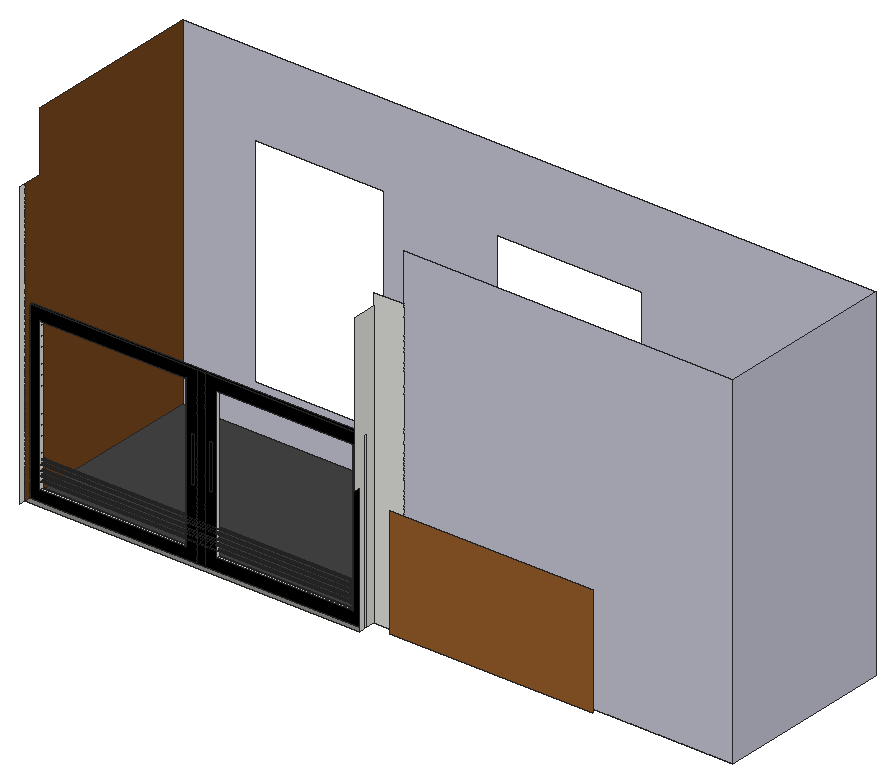
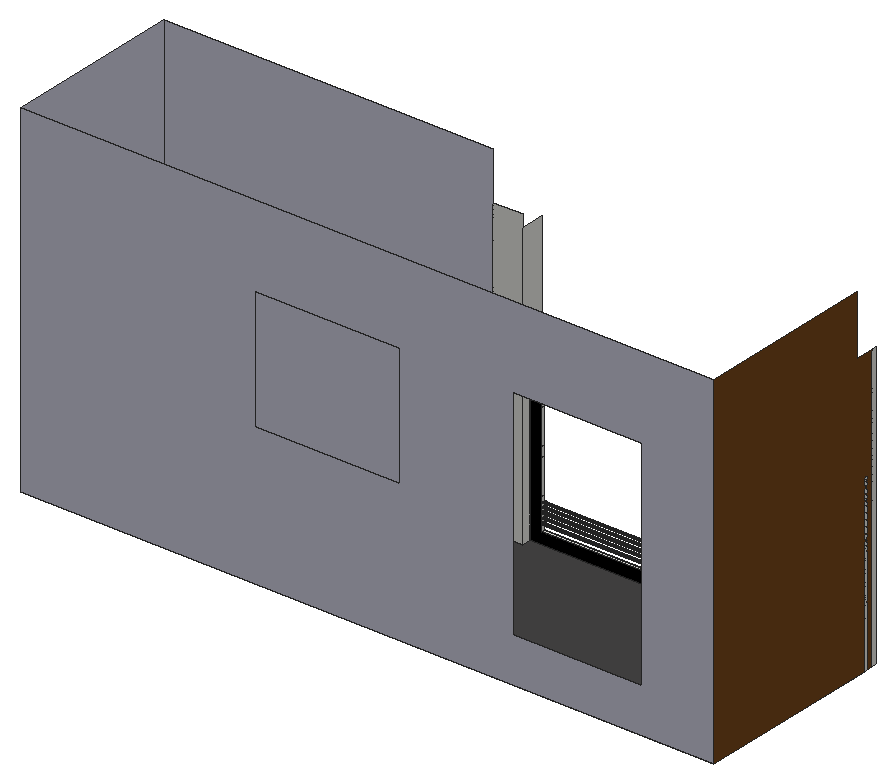
# SketchUp Ruby script. Lengths in inches.
U = 1.inch
M = Sketchup.active_model
def pt(a) = Geom::Point3d.new(a.map { |v| v * U })
def face(e, loops, mat)
  f = e.add_face(loops[0].map { |a| pt(a) })
  loops[1..].each { |l| e.add_face(l.map { |a| pt(a) }).erase! }
  f.material = f.back_material = mat if mat
  f
end
# faces: each face lists its corners as indices into pts; further lists are holes
def faces(e, pts, list, mat = nil) = list.each { |f| face(e, (f[0].is_a?(Array) ? f : [f]).map { |l| l.map { |i| pts[i] } }, mat) }
# xy, xz, yz: faces in a plane at the given z, y or x. An outline is a flat list of corners, or four numbers for a rectangle; further outlines are holes
def ring(l) = l.size == 4 ? [[l[0], l[1]], [l[2], l[1]], [l[2], l[3]], [l[0], l[3]]] : l.each_slice(2).to_a
def flat(e, list, mat, &to3) = list.each { |f| face(e, (f[0].is_a?(Array) ? f : [f]).map { |l| ring(l).map { |u, v| to3.(u, v) } }, mat) }
def xy(e, z, list, mat = nil) = flat(e, list, mat) { |x, y| [x, y, z] }
def xz(e, y, list, mat = nil) = flat(e, list, mat) { |x, z| [x, y, z] }
def yz(e, x, list, mat = nil) = flat(e, list, mat) { |y, z| [x, y, z] }
def lines(e, pts, list) = list.each { |a, b| e.add_line(pt(pts[a]), pt(pts[b])) }
# prism: a flat outline (further loops are holes) pulled along v
def prism(e, loops, v, mat = nil)
  f = face(e, loops, mat); d = Geom::Vector3d.new(v.map { |x| x * U })
  f.pushpull(f.normal.samedirection?(d) ? d.length : -d.length)
end
def box(e, o, s, mat = nil) = prism(e, [[o, [o[0] + s[0], o[1], o[2]], [o[0] + s[0], o[1] + s[1], o[2]], [o[0], o[1] + s[1], o[2]]]], [0, 0, s[2]], mat)
def at(x, y, z, deg = 0) = Geom::Transformation.translation(pt([x, y, z])) * Geom::Transformation.rotation(ORIGIN, Z_AXIS, deg.degrees)
def axes(o, x, y, z) = Geom::Transformation.new([*x, 0, *y, 0, *z, 0, *pt(o).to_a, 1])
def part(name) = M.definitions.add(name)
# library, detail: a bought-in or finely detailed component or shape, given as its bounding box
def library(name, o, s) = part(name).tap { |d| box(d.entities, o, s) }
def detail(e, o, s) = box(e.add_group.entities, o, s)
def put(e, d, t, mat = nil) = e.add_instance(d, t).tap { |i| i.material = mat if mat }
def group(e, t, mat = nil) = e.add_group.tap { |g| g.transformation = t; g.material = mat if mat }.entities
root = M.entities
M.materials.add("[0116_Lavender]").color = [199, 199, 216]
M.materials.add("[0137_Black]").color = [0, 0, 0]
M.materials.add("[Granite Dark Gray]").color = [69, 68, 68]
M.materials.add("[Granite Light Gray]").color = [132, 131, 128]
M.materials.add("[Wood Bamboo]").color = [114, 68, 27]
M.materials.add("[Wood Floor Dark]").color = [153, 94, 42]
xy(root,42,[[468,71.03,1140,78]])
xy(root,42,[[468,78,1140,78,1140,96,1860,96,1860,455.71,468,455.71]],"[Granite Dark Gray]")
xy(root,42,[[468,60,1140,71.03]],"[Granite Light Gray]")
xy(root,63.6,[[489.6,71.03,782.4,78]])
xy(root,65.95,[[843.34,71.03,1116.05,78]])
xz(root,60,[[1200,60,1608,280.8]],"[Wood Floor Dark]")
xz(root,71.03,[[[468,42,804,390],[489.6,63.6,782.4,368.4],[791.39,180.6,799.64,271.47]],[804,42,819.39,390],[[819.39,42,1140,390],[843.34,65.95,1116.05,366.05],[827.39,180.6,835.64,271.47]]],"[0137_Black]")
xz(root,78,[[[468,42,1140,390],[489.6,63.6,782.4,368.4],[843.34,65.95,1116.05,366.05]]],"[0137_Black]")
xz(root,96,[[1140,42,1200,636]])
xz(root,96,[[1200,42,1860,732]],"[0116_Lavender]")
xz(root,455.71,[[[468,42,1860,732],[611.72,132,872.28,567.56],[1098.44,324.3,1390.19,567.56]]],"[0116_Lavender]")
yz(root,468,[[48,42,60,612],[71.03,42,78,390]])
yz(root,468,[[60,42,71.03,42,71.03,390,78,390,78,42,455.71,42,455.71,732,96,732,96,612,60,612]],"[Wood Bamboo]")
yz(root,489.6,[[[71.03,63.6,78,368.4],[74.52,356.6875,74,356.75,73.52,356.95,73.1,357.27,72.78,357.6875,72.58,358.17,72.52,358.6875,72.58,359.2,72.78,359.6875,73.1,360.1,73.52,360.42,74,360.62,74.52,360.6875,75.03,360.62,75.52,360.42,75.93,360.1,76.25,359.6875,76.45,359.2,76.52,358.6875,76.45,358.17,76.25,357.6875,75.93,357.27,75.52,356.95,75.03,356.75],[74.52,346.6875,74,346.75,73.52,346.95,73.1,347.27,72.78,347.6875,72.58,348.17,72.52,348.6875,72.58,349.2,72.78,349.6875,73.1,350.1,73.52,350.42,74,350.62,74.52,350.6875,75.03,350.62,75.52,350.42,75.93,350.1,76.25,349.6875,76.45,349.2,76.52,348.6875,76.45,348.17,76.25,347.6875,75.93,347.27,75.52,346.95,75.03,346.75],[74.52,336.6875,74,336.75,73.52,336.95,73.1,337.27,72.78,337.6875,72.58,338.17,72.52,338.6875,72.58,339.2,72.78,339.6875,73.1,340.1,73.52,340.42,74,340.62,74.52,340.6875,75.03,340.62,75.52,340.42,75.93,340.1,76.25,339.6875,76.45,339.2,76.52,338.6875,76.45,338.17,76.25,337.6875,75.93,337.27,75.52,336.95,75.03,336.75],[74.52,326.6875,74,326.75,73.52,326.95,73.1,327.27,72.78,327.6875,72.58,328.17,72.52,328.6875,72.58,329.2,72.78,329.6875,73.1,330.1,73.52,330.42,74,330.62,74.52,330.6875,75.03,330.62,75.52,330.42,75.93,330.1,76.25,329.6875,76.45,329.2,76.52,328.6875,76.45,328.17,76.25,327.6875,75.93,327.27,75.52,326.95,75.03,326.75],[74.52,316.6875,74,316.75,73.52,316.95,73.1,317.27,72.78,317.6875,72.58,318.17,72.52,318.6875,72.58,319.2,72.78,319.6875,73.1,320.1,73.52,320.42,74,320.62,74.52,320.6875,75.03,320.62,75.52,320.42,75.93,320.1,76.25,319.6875,76.45,319.2,76.52,318.6875,76.45,318.17,76.25,317.6875,75.93,317.27,75.52,316.95,75.03,316.75],[74.52,306.6875,74,306.75,73.52,306.95,73.1,307.27,72.78,307.6875,72.58,308.17,72.52,308.6875,72.58,309.2,72.78,309.6875,73.1,310.1,73.52,310.42,74,310.62,74.52,310.6875,75.03,310.62,75.52,310.42,75.93,310.1,76.25,309.6875,76.45,309.2,76.52,308.6875,76.45,308.17,76.25,307.6875,75.93,307.27,75.52,306.95,75.03,306.75],[74.52,296.6875,74,296.75,73.52,296.95,73.1,297.27,72.78,297.6875,72.58,298.17,72.52,298.6875,72.58,299.2,72.78,299.6875,73.1,300.1,73.52,300.42,74,300.62,74.52,300.6875,75.03,300.62,75.52,300.42,75.93,300.1,76.25,299.6875,76.45,299.2,76.52,298.6875,76.45,298.17,76.25,297.6875,75.93,297.27,75.52,296.95,75.03,296.75],[74.52,286.6875,74,286.75,73.52,286.95,73.1,287.27,72.78,287.6875,72.58,288.17,72.52,288.6875,72.58,289.2,72.78,289.6875,73.1,290.1,73.52,290.42,74,290.62,74.52,290.6875,75.03,290.62,75.52,290.42,75.93,290.1,76.25,289.6875,76.45,289.2,76.52,288.6875,76.45,288.17,76.25,287.6875,75.93,287.27,75.52,286.95,75.03,286.75],[74.52,276.6875,74,276.75,73.52,276.95,73.1,277.27,72.78,277.6875,72.58,278.17,72.52,278.6875,72.58,279.2,72.78,279.6875,73.1,280.1,73.52,280.42,74,280.62,74.52,280.6875,75.03,280.62,75.52,280.42,75.93,280.1,76.25,279.6875,76.45,279.2,76.52,278.6875,76.45,278.17,76.25,277.6875,75.93,277.27,75.52,276.95,75.03,276.75],[74.52,266.6875,74,266.75,73.52,266.95,73.1,267.27,72.78,267.6875,72.58,268.17,72.52,268.6875,72.58,269.2,72.78,269.6875,73.1,270.1,73.52,270.42,74,270.62,74.52,270.6875,75.03,270.62,75.52,270.42,75.93,270.1,76.25,269.6875,76.45,269.2,76.52,268.6875,76.45,268.17,76.25,267.6875,75.93,267.27,75.52,266.95,75.03,266.75],[74.52,256.6875,74,256.75,73.52,256.95,73.1,257.27,72.78,257.6875,72.58,258.17,72.52,258.6875,72.58,259.2,72.78,259.6875,73.1,260.1,73.52,260.42,74,260.62,74.52,260.6875,75.03,260.62,75.52,260.42,75.93,260.1,76.25,259.6875,76.45,259.2,76.52,258.6875,76.45,258.17,76.25,257.6875,75.93,257.27,75.52,256.95,75.03,256.75],[74.52,246.6875,74,246.75,73.52,246.95,73.1,247.27,72.78,247.6875,72.58,248.17,72.52,248.6875,72.58,249.2,72.78,249.6875,73.1,250.1,73.52,250.42,74,250.62,74.52,250.6875,75.03,250.62,75.52,250.42,75.93,250.1,76.25,249.6875,76.45,249.2,76.52,248.6875,76.45,248.17,76.25,247.6875,75.93,247.27,75.52,246.95,75.03,246.75],[74.52,236.6875,74,236.75,73.52,236.95,73.1,237.27,72.78,237.6875,72.58,238.17,72.52,238.6875,72.58,239.2,72.78,239.6875,73.1,240.1,73.52,240.42,74,240.62,74.52,240.6875,75.03,240.62,75.52,240.42,75.93,240.1,76.25,239.6875,76.45,239.2,76.52,238.6875,76.45,238.17,76.25,237.6875,75.93,237.27,75.52,236.95,75.03,236.75],[74.52,226.6875,74,226.75,73.52,226.95,73.1,227.27,72.78,227.6875,72.58,228.17,72.52,228.6875,72.58,229.2,72.78,229.6875,73.1,230.1,73.52,230.42,74,230.62,74.52,230.6875,75.03,230.62,75.52,230.42,75.93,230.1,76.25,229.6875,76.45,229.2,76.52,228.6875,76.45,228.17,76.25,227.6875,75.93,227.27,75.52,226.95,75.03,226.75],[74.52,216.6875,74,216.75,73.52,216.95,73.1,217.27,72.78,217.6875,72.58,218.17,72.52,218.6875,72.58,219.2,72.78,219.6875,73.1,220.1,73.52,220.42,74,220.62,74.52,220.6875,75.03,220.62,75.52,220.42,75.93,220.1,76.25,219.6875,76.45,219.2,76.52,218.6875,76.45,218.17,76.25,217.6875,75.93,217.27,75.52,216.95,75.03,216.75],[74.52,206.6875,74,206.75,73.52,206.95,73.1,207.27,72.78,207.6875,72.58,208.17,72.52,208.6875,72.58,209.2,72.78,209.6875,73.1,210.1,73.52,210.42,74,210.62,74.52,210.6875,75.03,210.62,75.52,210.42,75.93,210.1,76.25,209.6875,76.45,209.2,76.52,208.6875,76.45,208.17,76.25,207.6875,75.93,207.27,75.52,206.95,75.03,206.75],[74.52,196.6875,74,196.75,73.52,196.95,73.1,197.27,72.78,197.6875,72.58,198.17,72.52,198.6875,72.58,199.2,72.78,199.6875,73.1,200.1,73.52,200.42,74,200.62,74.52,200.6875,75.03,200.62,75.52,200.42,75.93,200.1,76.25,199.6875,76.45,199.2,76.52,198.6875,76.45,198.17,76.25,197.6875,75.93,197.27,75.52,196.95,75.03,196.75],[74.52,186.6875,74,186.75,73.52,186.95,73.1,187.27,72.78,187.6875,72.58,188.17,72.52,188.6875,72.58,189.2,72.78,189.6875,73.1,190.1,73.52,190.42,74,190.62,74.52,190.6875,75.03,190.62,75.52,190.42,75.93,190.1,76.25,189.6875,76.45,189.2,76.52,188.6875,76.45,188.17,76.25,187.6875,75.93,187.27,75.52,186.95,75.03,186.75],[74.52,176.6875,74,176.75,73.52,176.95,73.1,177.27,72.78,177.6875,72.58,178.17,72.52,178.6875,72.58,179.2,72.78,179.6875,73.1,180.1,73.52,180.42,74,180.62,74.52,180.6875,75.03,180.62,75.52,180.42,75.93,180.1,76.25,179.6875,76.45,179.2,76.52,178.6875,76.45,178.17,76.25,177.6875,75.93,177.27,75.52,176.95,75.03,176.75],[74.52,166.6875,74,166.75,73.52,166.95,73.1,167.27,72.78,167.6875,72.58,168.17,72.52,168.6875,72.58,169.2,72.78,169.6875,73.1,170.1,73.52,170.42,74,170.62,74.52,170.6875,75.03,170.62,75.52,170.42,75.93,170.1,76.25,169.6875,76.45,169.2,76.52,168.6875,76.45,168.17,76.25,167.6875,75.93,167.27,75.52,166.95,75.03,166.75],[74.52,156.6875,74,156.75,73.52,156.95,73.1,157.27,72.78,157.6875,72.58,158.17,72.52,158.6875,72.58,159.2,72.78,159.6875,73.1,160.1,73.52,160.42,74,160.62,74.52,160.6875,75.03,160.62,75.52,160.42,75.93,160.1,76.25,159.6875,76.45,159.2,76.52,158.6875,76.45,158.17,76.25,157.6875,75.93,157.27,75.52,156.95,75.03,156.75],[74.52,146.6875,74,146.75,73.52,146.95,73.1,147.27,72.78,147.6875,72.58,148.17,72.52,148.6875,72.58,149.2,72.78,149.6875,73.1,150.1,73.52,150.42,74,150.62,74.52,150.6875,75.03,150.62,75.52,150.42,75.93,150.1,76.25,149.6875,76.45,149.2,76.52,148.6875,76.45,148.17,76.25,147.6875,75.93,147.27,75.52,146.95,75.03,146.75],[74.52,136.6875,74,136.75,73.52,136.95,73.1,137.27,72.78,137.6875,72.58,138.17,72.52,138.6875,72.58,139.2,72.78,139.6875,73.1,140.1,73.52,140.42,74,140.62,74.52,140.6875,75.03,140.62,75.52,140.42,75.93,140.1,76.25,139.6875,76.45,139.2,76.52,138.6875,76.45,138.17,76.25,137.6875,75.93,137.27,75.52,136.95,75.03,136.75],[74.52,126.6875,74,126.75,73.52,126.95,73.1,127.27,72.78,127.6875,72.58,128.17,72.52,128.6875,72.58,129.2,72.78,129.6875,73.1,130.1,73.52,130.42,74,130.62,74.52,130.6875,75.03,130.62,75.52,130.42,75.93,130.1,76.25,129.6875,76.45,129.2,76.52,128.6875,76.45,128.17,76.25,127.6875,75.93,127.27,75.52,126.95,75.03,126.75],[74.52,116.6875,74,116.75,73.52,116.95,73.1,117.27,72.78,117.6875,72.58,118.17,72.52,118.6875,72.58,119.2,72.78,119.6875,73.1,120.1,73.52,120.42,74,120.62,74.52,120.6875,75.03,120.62,75.52,120.42,75.93,120.1,76.25,119.6875,76.45,119.2,76.52,118.6875,76.45,118.17,76.25,117.6875,75.93,117.27,75.52,116.95,75.03,116.75],[74.52,106.6875,74,106.75,73.52,106.95,73.1,107.27,72.78,107.6875,72.58,108.17,72.52,108.6875,72.58,109.2,72.78,109.6875,73.1,110.1,73.52,110.42,74,110.62,74.52,110.6875,75.03,110.62,75.52,110.42,75.93,110.1,76.25,109.6875,76.45,109.2,76.52,108.6875,76.45,108.17,76.25,107.6875,75.93,107.27,75.52,106.95,75.03,106.75],[74.52,96.6875,74,96.75,73.52,96.95,73.1,97.27,72.78,97.6875,72.58,98.17,72.52,98.6875,72.58,99.2,72.78,99.6875,73.1,100.1,73.52,100.42,74,100.62,74.52,100.6875,75.03,100.62,75.52,100.42,75.93,100.1,76.25,99.6875,76.45,99.2,76.52,98.6875,76.45,98.17,76.25,97.6875,75.93,97.27,75.52,96.95,75.03,96.75],[74.52,86.6875,74,86.75,73.52,86.95,73.1,87.27,72.78,87.6875,72.58,88.17,72.52,88.6875,72.58,89.2,72.78,89.6875,73.1,90.1,73.52,90.42,74,90.62,74.52,90.6875,75.03,90.62,75.52,90.42,75.93,90.1,76.25,89.6875,76.45,89.2,76.52,88.6875,76.45,88.17,76.25,87.6875,75.93,87.27,75.52,86.95,75.03,86.75],[74.52,76.6875,74,76.75,73.52,76.95,73.1,77.27,72.78,77.6875,72.58,78.17,72.52,78.6875,72.58,79.2,72.78,79.6875,73.1,80.1,73.52,80.42,74,80.62,74.52,80.6875,75.03,80.62,75.52,80.42,75.93,80.1,76.25,79.6875,76.45,79.2,76.52,78.6875,76.45,78.17,76.25,77.6875,75.93,77.27,75.52,76.95,75.03,76.75]]])
yz(root,782.4,[[71.03,63.6,78,368.4]])
yz(root,843.34,[[71.03,65.95,78,366.05]])
yz(root,1116.05,[[[71.03,65.95,78,366.05],[74.52,316.6875,75.03,316.75,75.52,316.95,75.93,317.27,76.25,317.6875,76.45,318.17,76.52,318.6875,76.45,319.2,76.25,319.6875,75.93,320.1,75.52,320.42,75.03,320.62,74.52,320.6875,74,320.62,73.52,320.42,73.1,320.1,72.78,319.6875,72.58,319.2,72.52,318.6875,72.58,318.17,72.78,317.6875,73.1,317.27,73.52,316.95,74,316.75],[74.52,326.6875,75.03,326.75,75.52,326.95,75.93,327.27,76.25,327.6875,76.45,328.17,76.52,328.6875,76.45,329.2,76.25,329.6875,75.93,330.1,75.52,330.42,75.03,330.62,74.52,330.6875,74,330.62,73.52,330.42,73.1,330.1,72.78,329.6875,72.58,329.2,72.52,328.6875,72.58,328.17,72.78,327.6875,73.1,327.27,73.52,326.95,74,326.75],[74.52,346.6875,75.03,346.75,75.52,346.95,75.93,347.27,76.25,347.6875,76.45,348.17,76.52,348.6875,76.45,349.2,76.25,349.6875,75.93,350.1,75.52,350.42,75.03,350.62,74.52,350.6875,74,350.62,73.52,350.42,73.1,350.1,72.78,349.6875,72.58,349.2,72.52,348.6875,72.58,348.17,72.78,347.6875,73.1,347.27,73.52,346.95,74,346.75],[74.52,356.6875,75.03,356.75,75.52,356.95,75.93,357.27,76.25,357.6875,76.45,358.17,76.52,358.6875,76.45,359.2,76.25,359.6875,75.93,360.1,75.52,360.42,75.03,360.62,74.52,360.6875,74,360.62,73.52,360.42,73.1,360.1,72.78,359.6875,72.58,359.2,72.52,358.6875,72.58,358.17,72.78,357.6875,73.1,357.27,73.52,356.95,74,356.75],[74.52,136.6875,75.03,136.75,75.52,136.95,75.93,137.27,76.25,137.6875,76.45,138.17,76.52,138.6875,76.45,139.2,76.25,139.6875,75.93,140.1,75.52,140.42,75.03,140.62,74.52,140.6875,74,140.62,73.52,140.42,73.1,140.1,72.78,139.6875,72.58,139.2,72.52,138.6875,72.58,138.17,72.78,137.6875,73.1,137.27,73.52,136.95,74,136.75],[74.52,146.6875,75.03,146.75,75.52,146.95,75.93,147.27,76.25,147.6875,76.45,148.17,76.52,148.6875,76.45,149.2,76.25,149.6875,75.93,150.1,75.52,150.42,75.03,150.62,74.52,150.6875,74,150.62,73.52,150.42,73.1,150.1,72.78,149.6875,72.58,149.2,72.52,148.6875,72.58,148.17,72.78,147.6875,73.1,147.27,73.52,146.95,74,146.75],[74.52,156.6875,75.03,156.75,75.52,156.95,75.93,157.27,76.25,157.6875,76.45,158.17,76.52,158.6875,76.45,159.2,76.25,159.6875,75.93,160.1,75.52,160.42,75.03,160.62,74.52,160.6875,74,160.62,73.52,160.42,73.1,160.1,72.78,159.6875,72.58,159.2,72.52,158.6875,72.58,158.17,72.78,157.6875,73.1,157.27,73.52,156.95,74,156.75],[74.52,166.6875,75.03,166.75,75.52,166.95,75.93,167.27,76.25,167.6875,76.45,168.17,76.52,168.6875,76.45,169.2,76.25,169.6875,75.93,170.1,75.52,170.42,75.03,170.62,74.52,170.6875,74,170.62,73.52,170.42,73.1,170.1,72.78,169.6875,72.58,169.2,72.52,168.6875,72.58,168.17,72.78,167.6875,73.1,167.27,73.52,166.95,74,166.75],[74.52,176.6875,75.03,176.75,75.52,176.95,75.93,177.27,76.25,177.6875,76.45,178.17,76.52,178.6875,76.45,179.2,76.25,179.6875,75.93,180.1,75.52,180.42,75.03,180.62,74.52,180.6875,74,180.62,73.52,180.42,73.1,180.1,72.78,179.6875,72.58,179.2,72.52,178.6875,72.58,178.17,72.78,177.6875,73.1,177.27,73.52,176.95,74,176.75],[74.52,186.6875,75.03,186.75,75.52,186.95,75.93,187.27,76.25,187.6875,76.45,188.17,76.52,188.6875,76.45,189.2,76.25,189.6875,75.93,190.1,75.52,190.42,75.03,190.62,74.52,190.6875,74,190.62,73.52,190.42,73.1,190.1,72.78,189.6875,72.58,189.2,72.52,188.6875,72.58,188.17,72.78,187.6875,73.1,187.27,73.52,186.95,74,186.75],[74.52,196.6875,75.03,196.75,75.52,196.95,75.93,197.27,76.25,197.6875,76.45,198.17,76.52,198.6875,76.45,199.2,76.25,199.6875,75.93,200.1,75.52,200.42,75.03,200.62,74.52,200.6875,74,200.62,73.52,200.42,73.1,200.1,72.78,199.6875,72.58,199.2,72.52,198.6875,72.58,198.17,72.78,197.6875,73.1,197.27,73.52,196.95,74,196.75],[74.52,206.6875,75.03,206.75,75.52,206.95,75.93,207.27,76.25,207.6875,76.45,208.17,76.52,208.6875,76.45,209.2,76.25,209.6875,75.93,210.1,75.52,210.42,75.03,210.62,74.52,210.6875,74,210.62,73.52,210.42,73.1,210.1,72.78,209.6875,72.58,209.2,72.52,208.6875,72.58,208.17,72.78,207.6875,73.1,207.27,73.52,206.95,74,206.75],[74.52,216.6875,75.03,216.75,75.52,216.95,75.93,217.27,76.25,217.6875,76.45,218.17,76.52,218.6875,76.45,219.2,76.25,219.6875,75.93,220.1,75.52,220.42,75.03,220.62,74.52,220.6875,74,220.62,73.52,220.42,73.1,220.1,72.78,219.6875,72.58,219.2,72.52,218.6875,72.58,218.17,72.78,217.6875,73.1,217.27,73.52,216.95,74,216.75],[74.52,226.6875,75.03,226.75,75.52,226.95,75.93,227.27,76.25,227.6875,76.45,228.17,76.52,228.6875,76.45,229.2,76.25,229.6875,75.93,230.1,75.52,230.42,75.03,230.62,74.52,230.6875,74,230.62,73.52,230.42,73.1,230.1,72.78,229.6875,72.58,229.2,72.52,228.6875,72.58,228.17,72.78,227.6875,73.1,227.27,73.52,226.95,74,226.75],[74.52,236.6875,75.03,236.75,75.52,236.95,75.93,237.27,76.25,237.6875,76.45,238.17,76.52,238.6875,76.45,239.2,76.25,239.6875,75.93,240.1,75.52,240.42,75.03,240.62,74.52,240.6875,74,240.62,73.52,240.42,73.1,240.1,72.78,239.6875,72.58,239.2,72.52,238.6875,72.58,238.17,72.78,237.6875,73.1,237.27,73.52,236.95,74,236.75],[74.52,246.6875,75.03,246.75,75.52,246.95,75.93,247.27,76.25,247.6875,76.45,248.17,76.52,248.6875,76.45,249.2,76.25,249.6875,75.93,250.1,75.52,250.42,75.03,250.62,74.52,250.6875,74,250.62,73.52,250.42,73.1,250.1,72.78,249.6875,72.58,249.2,72.52,248.6875,72.58,248.17,72.78,247.6875,73.1,247.27,73.52,246.95,74,246.75],[74.52,256.6875,75.03,256.75,75.52,256.95,75.93,257.27,76.25,257.6875,76.45,258.17,76.52,258.6875,76.45,259.2,76.25,259.6875,75.93,260.1,75.52,260.42,75.03,260.62,74.52,260.6875,74,260.62,73.52,260.42,73.1,260.1,72.78,259.6875,72.58,259.2,72.52,258.6875,72.58,258.17,72.78,257.6875,73.1,257.27,73.52,256.95,74,256.75],[74.52,266.6875,75.03,266.75,75.52,266.95,75.93,267.27,76.25,267.6875,76.45,268.17,76.52,268.6875,76.45,269.2,76.25,269.6875,75.93,270.1,75.52,270.42,75.03,270.62,74.52,270.6875,74,270.62,73.52,270.42,73.1,270.1,72.78,269.6875,72.58,269.2,72.52,268.6875,72.58,268.17,72.78,267.6875,73.1,267.27,73.52,266.95,74,266.75],[74.52,276.6875,75.03,276.75,75.52,276.95,75.93,277.27,76.25,277.6875,76.45,278.17,76.52,278.6875,76.45,279.2,76.25,279.6875,75.93,280.1,75.52,280.42,75.03,280.62,74.52,280.6875,74,280.62,73.52,280.42,73.1,280.1,72.78,279.6875,72.58,279.2,72.52,278.6875,72.58,278.17,72.78,277.6875,73.1,277.27,73.52,276.95,74,276.75],[74.52,286.6875,75.03,286.75,75.52,286.95,75.93,287.27,76.25,287.6875,76.45,288.17,76.52,288.6875,76.45,289.2,76.25,289.6875,75.93,290.1,75.52,290.42,75.03,290.62,74.52,290.6875,74,290.62,73.52,290.42,73.1,290.1,72.78,289.6875,72.58,289.2,72.52,288.6875,72.58,288.17,72.78,287.6875,73.1,287.27,73.52,286.95,74,286.75],[74.52,296.6875,75.03,296.75,75.52,296.95,75.93,297.27,76.25,297.6875,76.45,298.17,76.52,298.6875,76.45,299.2,76.25,299.6875,75.93,300.1,75.52,300.42,75.03,300.62,74.52,300.6875,74,300.62,73.52,300.42,73.1,300.1,72.78,299.6875,72.58,299.2,72.52,298.6875,72.58,298.17,72.78,297.6875,73.1,297.27,73.52,296.95,74,296.75],[74.52,306.6875,75.03,306.75,75.52,306.95,75.93,307.27,76.25,307.6875,76.45,308.17,76.52,308.6875,76.45,309.2,76.25,309.6875,75.93,310.1,75.52,310.42,75.03,310.62,74.52,310.6875,74,310.62,73.52,310.42,73.1,310.1,72.78,309.6875,72.58,309.2,72.52,308.6875,72.58,308.17,72.78,307.6875,73.1,307.27,73.52,306.95,74,306.75],[74.52,126.6875,75.03,126.75,75.52,126.95,75.93,127.27,76.25,127.6875,76.45,128.17,76.52,128.6875,76.45,129.2,76.25,129.6875,75.93,130.1,75.52,130.42,75.03,130.62,74.52,130.6875,74,130.62,73.52,130.42,73.1,130.1,72.78,129.6875,72.58,129.2,72.52,128.6875,72.58,128.17,72.78,127.6875,73.1,127.27,73.52,126.95,74,126.75],[74.52,76.6875,75.03,76.75,75.52,76.95,75.93,77.27,76.25,77.6875,76.45,78.17,76.52,78.6875,76.45,79.2,76.25,79.6875,75.93,80.1,75.52,80.42,75.03,80.62,74.52,80.6875,74,80.62,73.52,80.42,73.1,80.1,72.78,79.6875,72.58,79.2,72.52,78.6875,72.58,78.17,72.78,77.6875,73.1,77.27,73.52,76.95,74,76.75],[74.52,86.6875,75.03,86.75,75.52,86.95,75.93,87.27,76.25,87.6875,76.45,88.17,76.52,88.6875,76.45,89.2,76.25,89.6875,75.93,90.1,75.52,90.42,75.03,90.62,74.52,90.6875,74,90.62,73.52,90.42,73.1,90.1,72.78,89.6875,72.58,89.2,72.52,88.6875,72.58,88.17,72.78,87.6875,73.1,87.27,73.52,86.95,74,86.75],[74.52,96.6875,75.03,96.75,75.52,96.95,75.93,97.27,76.25,97.6875,76.45,98.17,76.52,98.6875,76.45,99.2,76.25,99.6875,75.93,100.1,75.52,100.42,75.03,100.62,74.52,100.6875,74,100.62,73.52,100.42,73.1,100.1,72.78,99.6875,72.58,99.2,72.52,98.6875,72.58,98.17,72.78,97.6875,73.1,97.27,73.52,96.95,74,96.75],[74.52,106.6875,75.03,106.75,75.52,106.95,75.93,107.27,76.25,107.6875,76.45,108.17,76.52,108.6875,76.45,109.2,76.25,109.6875,75.93,110.1,75.52,110.42,75.03,110.62,74.52,110.6875,74,110.62,73.52,110.42,73.1,110.1,72.78,109.6875,72.58,109.2,72.52,108.6875,72.58,108.17,72.78,107.6875,73.1,107.27,73.52,106.95,74,106.75]]])
yz(root,1116.35,[[74.52,116.6875,75.03,116.75,75.52,116.95,75.93,117.27,76.25,117.6875,76.45,118.17,76.52,118.6875,76.45,119.2,76.25,119.6875,75.93,120.1,75.52,120.42,75.03,120.62,74.52,120.6875,74,120.62,73.52,120.42,73.1,120.1,72.78,119.6875,72.58,119.2,72.52,118.6875,72.58,118.17,72.78,117.6875,73.1,117.27,73.52,116.95,74,116.75]])
yz(root,1140,[[60,42,60,300,48,300,48,612,96,612,96,42,78,42,78,390,71.03,390,71.03,42],[71.03,42,78,390]])
yz(root,1860,[[96,42,455.71,732]],"[0116_Lavender]")
p = [[489.6,74,76.75],[489.6,74.52,76.6875],[1116.05,74.52,76.6875],[1116.05,74,76.75],[489.6,75.03,76.75],[1116.05,75.03,76.75],
  [489.6,73.52,76.95],[1116.05,73.52,76.95],[489.6,75.52,76.95],[1116.05,75.52,76.95],[489.6,73.1,77.27],[1116.05,73.1,77.27],
  [489.6,75.93,77.27],[1116.05,75.93,77.27],[489.6,72.78,77.6875],[1116.05,72.78,77.6875],[489.6,76.25,77.6875],[1116.05,76.25,77.6875],
  [489.6,72.58,78.17],[1116.05,72.58,78.17],[489.6,76.45,78.17],[1116.05,76.45,78.17],[489.6,72.52,78.6875],[1116.05,72.52,78.6875],
  [489.6,76.52,78.6875],[1116.05,76.52,78.6875],[489.6,72.58,79.2],[1116.05,72.58,79.2],[489.6,76.45,79.2],[1116.05,76.45,79.2],
  [489.6,72.78,79.6875],[1116.05,72.78,79.6875],[489.6,76.25,79.6875],[1116.05,76.25,79.6875],[489.6,73.1,80.1],[1116.05,73.1,80.1],
  [489.6,75.93,80.1],[1116.05,75.93,80.1],[489.6,73.52,80.42],[1116.05,73.52,80.42],[489.6,75.52,80.42],[1116.05,75.52,80.42],
  [489.6,74,80.62],[1116.05,74,80.62],[489.6,75.03,80.62],[1116.05,75.03,80.62],[489.6,74.52,80.6875],[1116.05,74.52,80.6875],
  [489.6,74,86.75],[489.6,74.52,86.6875],[1116.05,74.52,86.6875],[1116.05,74,86.75],[489.6,75.03,86.75],[1116.05,75.03,86.75],
  [489.6,73.52,86.95],[1116.05,73.52,86.95],[489.6,75.52,86.95],[1116.05,75.52,86.95],[489.6,73.1,87.27],[1116.05,73.1,87.27],
  [489.6,75.93,87.27],[1116.05,75.93,87.27],[489.6,72.78,87.6875],[1116.05,72.78,87.6875],[489.6,76.25,87.6875],[1116.05,76.25,87.6875],
  [489.6,72.58,88.17],[1116.05,72.58,88.17],[489.6,76.45,88.17],[1116.05,76.45,88.17],[489.6,72.52,88.6875],[1116.05,72.52,88.6875],
  [489.6,76.52,88.6875],[1116.05,76.52,88.6875],[489.6,72.58,89.2],[1116.05,72.58,89.2],[489.6,76.45,89.2],[1116.05,76.45,89.2],
  [489.6,72.78,89.6875],[1116.05,72.78,89.6875],[489.6,76.25,89.6875],[1116.05,76.25,89.6875],[489.6,73.1,90.1],[1116.05,73.1,90.1],
  [489.6,75.93,90.1],[1116.05,75.93,90.1],[489.6,73.52,90.42],[1116.05,73.52,90.42],[489.6,75.52,90.42],[1116.05,75.52,90.42],
  [489.6,74,90.62],[1116.05,74,90.62],[489.6,75.03,90.62],[1116.05,75.03,90.62],[489.6,74.52,90.6875],[1116.05,74.52,90.6875],
  [489.6,74,96.75],[489.6,74.52,96.6875],[1116.05,74.52,96.6875],[1116.05,74,96.75],[489.6,75.03,96.75],[1116.05,75.03,96.75],
  [489.6,73.52,96.95],[1116.05,73.52,96.95],[489.6,75.52,96.95],[1116.05,75.52,96.95],[489.6,73.1,97.27],[1116.05,73.1,97.27],
  [489.6,75.93,97.27],[1116.05,75.93,97.27],[489.6,72.78,97.6875],[1116.05,72.78,97.6875],[489.6,76.25,97.6875],[1116.05,76.25,97.6875],
  [489.6,72.58,98.17],[1116.05,72.58,98.17],[489.6,76.45,98.17],[1116.05,76.45,98.17],[489.6,72.52,98.6875],[1116.05,72.52,98.6875],
  [489.6,76.52,98.6875],[1116.05,76.52,98.6875],[489.6,72.58,99.2],[1116.05,72.58,99.2],[489.6,76.45,99.2],[1116.05,76.45,99.2],
  [489.6,72.78,99.6875],[1116.05,72.78,99.6875],[489.6,76.25,99.6875],[1116.05,76.25,99.6875],[489.6,73.1,100.1],[1116.05,73.1,100.1],
  [489.6,75.93,100.1],[1116.05,75.93,100.1],[489.6,73.52,100.42],[1116.05,73.52,100.42],[489.6,75.52,100.42],[1116.05,75.52,100.42],
  [489.6,74,100.62],[1116.05,74,100.62],[489.6,75.03,100.62],[1116.05,75.03,100.62],[489.6,74.52,100.6875],[1116.05,74.52,100.6875],
  [489.6,74,106.75],[489.6,74.52,106.6875],[1116.05,74.52,106.6875],[1116.05,74,106.75],[489.6,75.03,106.75],[1116.05,75.03,106.75],
  [489.6,73.52,106.95],[1116.05,73.52,106.95],[489.6,75.52,106.95],[1116.05,75.52,106.95],[489.6,73.1,107.27],[1116.05,73.1,107.27],
  [489.6,75.93,107.27],[1116.05,75.93,107.27],[489.6,72.78,107.6875],[1116.05,72.78,107.6875],[489.6,76.25,107.6875],[1116.05,76.25,107.6875],
  [489.6,72.58,108.17],[1116.05,72.58,108.17],[489.6,76.45,108.17],[1116.05,76.45,108.17],[489.6,72.52,108.6875],[1116.05,72.52,108.6875],
  [489.6,76.52,108.6875],[1116.05,76.52,108.6875],[489.6,72.58,109.2],[1116.05,72.58,109.2],[489.6,76.45,109.2],[1116.05,76.45,109.2],
  [489.6,72.78,109.6875],[1116.05,72.78,109.6875],[489.6,76.25,109.6875],[1116.05,76.25,109.6875],[489.6,73.1,110.1],[1116.05,73.1,110.1],
  [489.6,75.93,110.1],[1116.05,75.93,110.1],[489.6,73.52,110.42],[1116.05,73.52,110.42],[489.6,75.52,110.42],[1116.05,75.52,110.42],
  [489.6,74,110.62],[1116.05,74,110.62],[489.6,75.03,110.62],[1116.05,75.03,110.62],[489.6,74.52,110.6875],[1116.05,74.52,110.6875],
  [489.6,74,116.75],[489.6,74.52,116.6875],[1116.35,74.52,116.6875],[1116.35,74,116.75],[489.6,75.03,116.75],[1116.35,75.03,116.75],
  [489.6,73.52,116.95],[1116.35,73.52,116.95],[489.6,75.52,116.95],[1116.35,75.52,116.95],[489.6,73.1,117.27],[1116.35,73.1,117.27],
  [489.6,75.93,117.27],[1116.35,75.93,117.27],[489.6,72.78,117.6875],[1116.35,72.78,117.6875],[489.6,76.25,117.6875],[1116.35,76.25,117.6875],
  [489.6,72.58,118.17],[1116.35,72.58,118.17],[489.6,76.45,118.17],[1116.35,76.45,118.17],[489.6,72.52,118.6875],[1116.35,72.52,118.6875],
  [489.6,76.52,118.6875],[1116.35,76.52,118.6875],[489.6,72.58,119.2],[1116.35,72.58,119.2],[489.6,76.45,119.2],[1116.35,76.45,119.2]]
faces(root,p,[[0,1,2,3],[1,4,5,2],[6,0,3,7],[4,8,9,5],[10,6,7,11],[8,12,13,9],[14,10,11,15],[12,16,17,13],
  [18,14,15,19],[16,20,21,17],[22,18,19,23],[20,24,25,21],[26,22,23,27],[24,28,29,25],[30,26,27,31],[28,32,33,29],
  [34,30,31,35],[32,36,37,33],[38,34,35,39],[36,40,41,37],[42,38,39,43],[40,44,45,41],[46,42,43,47],[44,46,47,45],
  [48,49,50,51],[49,52,53,50],[54,48,51,55],[52,56,57,53],[58,54,55,59],[56,60,61,57],[62,58,59,63],[60,64,65,61],
  [66,62,63,67],[64,68,69,65],[70,66,67,71],[68,72,73,69],[74,70,71,75],[72,76,77,73],[78,74,75,79],[76,80,81,77],
  [82,78,79,83],[80,84,85,81],[86,82,83,87],[84,88,89,85],[90,86,87,91],[88,92,93,89],[94,90,91,95],[92,94,95,93],
  [96,97,98,99],[97,100,101,98],[102,96,99,103],[100,104,105,101],[106,102,103,107],[104,108,109,105],[110,106,107,111],[108,112,113,109],
  [114,110,111,115],[112,116,117,113],[118,114,115,119],[116,120,121,117],[122,118,119,123],[120,124,125,121],[126,122,123,127],[124,128,129,125],
  [130,126,127,131],[128,132,133,129],[134,130,131,135],[132,136,137,133],[138,134,135,139],[136,140,141,137],[142,138,139,143],[140,142,143,141],
  [144,145,146,147],[145,148,149,146],[150,144,147,151],[148,152,153,149],[154,150,151,155],[152,156,157,153],[158,154,155,159],[156,160,161,157],
  [162,158,159,163],[160,164,165,161],[166,162,163,167],[164,168,169,165],[170,166,167,171],[168,172,173,169],[174,170,171,175],[172,176,177,173],
  [178,174,175,179],[176,180,181,177],[182,178,179,183],[180,184,185,181],[186,182,183,187],[184,188,189,185],[190,186,187,191],[188,190,191,189],
  [192,193,194,195],[193,196,197,194],[198,192,195,199],[196,200,201,197],[202,198,199,203],[200,204,205,201],[206,202,203,207],[204,208,209,205],
  [210,206,207,211],[208,212,213,209],[214,210,211,215],[212,216,217,213],[218,214,215,219],[216,220,221,217]])
